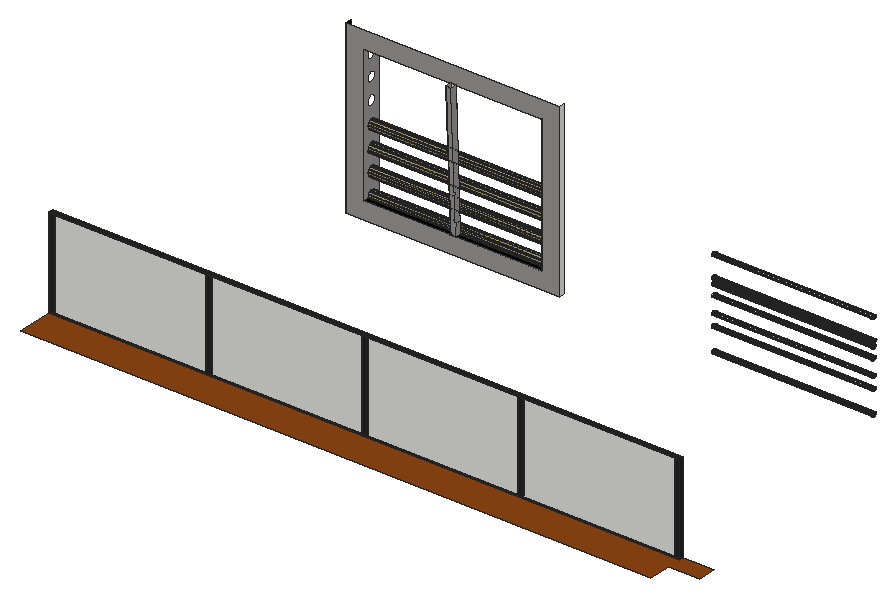
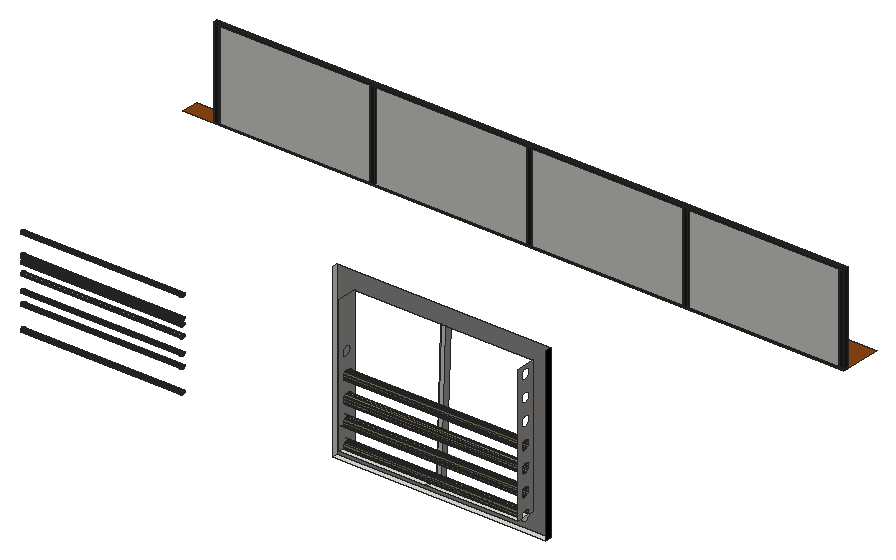
# SketchUp Ruby script. Lengths in inches.
U = 1.inch
M = Sketchup.active_model
def pt(a) = Geom::Point3d.new(a.map { |v| v * U })
def face(e, loops, mat)
  f = e.add_face(loops[0].map { |a| pt(a) })
  loops[1..].each { |l| e.add_face(l.map { |a| pt(a) }).erase! }
  f.material = f.back_material = mat if mat
  f
end
# faces: each face lists its corners as indices into pts; further lists are holes
def faces(e, pts, list, mat = nil) = list.each { |f| face(e, (f[0].is_a?(Array) ? f : [f]).map { |l| l.map { |i| pts[i] } }, mat) }
# xy, xz, yz: faces in a plane at the given z, y or x. An outline is a flat list of corners, or four numbers for a rectangle; further outlines are holes
def ring(l) = l.size == 4 ? [[l[0], l[1]], [l[2], l[1]], [l[2], l[3]], [l[0], l[3]]] : l.each_slice(2).to_a
def flat(e, list, mat, &to3) = list.each { |f| face(e, (f[0].is_a?(Array) ? f : [f]).map { |l| ring(l).map { |u, v| to3.(u, v) } }, mat) }
def xy(e, z, list, mat = nil) = flat(e, list, mat) { |x, y| [x, y, z] }
def xz(e, y, list, mat = nil) = flat(e, list, mat) { |x, z| [x, y, z] }
def yz(e, x, list, mat = nil) = flat(e, list, mat) { |y, z| [x, y, z] }
def lines(e, pts, list) = list.each { |a, b| e.add_line(pt(pts[a]), pt(pts[b])) }
# prism: a flat outline (further loops are holes) pulled along v
def prism(e, loops, v, mat = nil)
  f = face(e, loops, mat); d = Geom::Vector3d.new(v.map { |x| x * U })
  f.pushpull(f.normal.samedirection?(d) ? d.length : -d.length)
end
def box(e, o, s, mat = nil) = prism(e, [[o, [o[0] + s[0], o[1], o[2]], [o[0] + s[0], o[1] + s[1], o[2]], [o[0], o[1] + s[1], o[2]]]], [0, 0, s[2]], mat)
def at(x, y, z, deg = 0) = Geom::Transformation.translation(pt([x, y, z])) * Geom::Transformation.rotation(ORIGIN, Z_AXIS, deg.degrees)
def axes(o, x, y, z) = Geom::Transformation.new([*x, 0, *y, 0, *z, 0, *pt(o).to_a, 1])
def part(name) = M.definitions.add(name)
# library, detail: a bought-in or finely detailed component or shape, given as its bounding box
def library(name, o, s) = part(name).tap { |d| box(d.entities, o, s) }
def detail(e, o, s) = box(e.add_group.entities, o, s)
def put(e, d, t, mat = nil) = e.add_instance(d, t).tap { |i| i.material = mat if mat }
def group(e, t, mat = nil) = e.add_group.tap { |g| g.transformation = t; g.material = mat if mat }.entities
root = M.entities
M.materials.add("[0043_SaddleBrown]").color = [139, 69, 19]
M.materials.add("[0136_Charcoal]").color = [35, 35, 35]
M.materials.add("[Color M09]").color = [0, 0, 0]
M.materials.add("[Concrete Aggregate Smoke]").color = [154, 150, 148]
M.materials.add("[Terrazzo Tile Light]").color = [219, 217, 210]
M.materials.add("[Wood Lumber ButtJoined]").color = [164, 152, 112]
c1 = part("Group\#2")
box(c1.entities,[-152.36,0,0],[152.36,1.57,1.57])
c2 = part("Glass+Wall")
g1 = group(c2.entities,at(79.73,0,0))
g2 = group(g1,at(0,0,0))
g3 = group(g2,at(195.28,0,0),"[0136_Charcoal]")
box(g3,[-195.28,0,0],[195.28,1.57,1.57])
put(g2,c1,axes([1.57,0,116.54],[0,0,0.75452],[0,1,0],[-1,0,0]),"[0136_Charcoal]")
put(g2,c1,axes([50,0,116.54],[0,0,0.75452],[0,1,0],[-1,0,0]),"[0136_Charcoal]")
g4 = group(g2,at(195.28,0,115.75),"[0136_Charcoal]")
box(g4,[-195.28,0,0.79],[195.28,1.57,1.57])
put(g2,c1,axes([98.43,0,116.54],[0,0,0.75452],[0,1,0],[-1,0,0]),"[0136_Charcoal]")
put(g2,c1,axes([146.85,0,116.54],[0,0,0.75452],[0,1,0],[-1,0,0]),"[0136_Charcoal]")
put(g2,c1,axes([195.28,0,116.54],[0,0,0.75452],[0,1,0],[-1,0,0]),"[0136_Charcoal]")
g5 = group(g1,at(1.57,0.39,1.57))
box(g5,[0,0,0],[192.125,0.79,114.96])
xy(root,127.72,[[282.78,244.17,394.09,247.17]])
xy(root,136.72,[[291.78,246.86,291.78,251.79,338.43,251.79,338.43,247.17,339.9,247.17,339.9,251.79,385.09,251.79,385.09,246.86],[385.09,246.86,387.03,251.79],[338.43,247.17,339.9,251.79],[291.78,251.79,338.43,254.42],[338.43,251.79,339.9,254.42],
  [339.9,251.79,385.09,254.42]])
xy(root,136.72,[[291.78,244.17,385.09,246.86]],"[Color M09]")
xy(root,144,[[258.19,62.42,587.04,62.42,587.04,74.42,603,74.42,603,83.42,258.19,83.42]],"[0043_SaddleBrown]")
xz(root,244.17,[[[282.78,127.72,394.09,216.54],[291.78,136.72,385.09,207.54]]],"[Concrete Aggregate Smoke]")
yz(root,282.78,[[244.17,127.72,247.17,216.54]],"[Color M09]")
yz(root,291.78,[[249.32,134.85,249.99,134.94,250.6,135.2,251.14,135.6,251.54,136.13,251.79,136.72,246.86,136.72,247.1,136.13,247.51,135.6,248.04,135.2,248.66,134.94]])
yz(root,291.78,[[[244.17,136.72,246.86,136.72,246.85,136.75,246.76,137.42,246.85,138.08,247.1,138.7,247.51,139.23,248.04,139.63,248.66,139.89,249.32,139.98,249.99,139.89,250.6,139.63,251.14,139.23,251.54,138.7,251.8,138.08,251.89,137.42,251.8,136.75,251.79,136.72,254.42,136.72,254.42,207.54,244.17,207.54],[249.32,200.85,248.66,200.94,248.04,201.2,247.51,201.6,247.1,202.13,246.85,202.75,246.76,203.42,246.85,204.08,247.1,204.7,247.51,205.23,248.04,205.63,248.66,205.89,249.32,205.98,249.99,205.89,250.6,205.63,251.14,205.23,251.54,204.7,251.8,204.08,251.89,203.42,251.8,202.75,251.54,202.13,251.14,201.6,250.6,201.2,249.99,200.94],[249.32,189.85,248.66,189.94,248.04,190.2,247.51,190.6,247.1,191.13,246.85,191.75,246.76,192.42,246.85,193.08,247.1,193.7,247.51,194.23,248.04,194.63,248.66,194.89,249.32,194.98,249.99,194.89,250.6,194.63,251.14,194.23,251.54,193.7,251.8,193.08,251.89,192.42,251.8,191.75,251.54,191.13,251.14,190.6,250.6,190.2,249.99,189.94],[249.32,178.85,248.66,178.94,248.04,179.2,247.51,179.6,247.1,180.13,246.85,180.75,246.76,181.42,246.85,182.08,247.1,182.7,247.51,183.23,248.04,183.63,248.66,183.89,249.32,183.98,249.99,183.89,250.6,183.63,251.14,183.23,251.54,182.7,251.8,182.08,251.89,181.42,251.8,180.75,251.54,180.13,251.14,179.6,250.6,179.2,249.99,178.94],[249.32,167.85,248.66,167.94,248.04,168.2,247.51,168.6,247.1,169.13,246.85,169.75,246.76,170.42,246.85,171.08,247.1,171.7,247.51,172.23,248.04,172.63,248.66,172.89,249.32,172.98,249.99,172.89,250.6,172.63,251.14,172.23,251.54,171.7,251.8,171.08,251.89,170.42,251.8,169.75,251.54,169.13,251.14,168.6,250.6,168.2,249.99,167.94],[249.32,156.85,248.66,156.94,248.04,157.2,247.51,157.6,247.1,158.13,246.85,158.75,246.76,159.42,246.85,160.08,247.1,160.7,247.51,161.23,248.04,161.63,248.66,161.89,249.32,161.98,249.99,161.89,250.6,161.63,251.14,161.23,251.54,160.7,251.8,160.08,251.89,159.42,251.8,158.75,251.54,158.13,251.14,157.6,250.6,157.2,249.99,156.94],[249.32,145.85,248.66,145.94,248.04,146.2,247.51,146.6,247.1,147.13,246.85,147.75,246.76,148.42,246.85,149.08,247.1,149.7,247.51,150.23,248.04,150.63,248.66,150.89,249.32,150.98,249.99,150.89,250.6,150.63,251.14,150.23,251.54,149.7,251.8,149.08,251.89,148.42,251.8,147.75,251.54,147.13,251.14,146.6,250.6,146.2,249.99,145.94]]],"[Concrete Aggregate Smoke]")
yz(root,337.18,[[244.18,136.6,244.17,136.72,241.18,207.41,244.17,207.54,247.17,136.72]],"[Concrete Aggregate Smoke]")
yz(root,339.9,[[244.18,136.6,247.17,136.72,244.17,207.54,241.18,207.41,244.17,136.72]],"[Concrete Aggregate Smoke]")
yz(root,385.09,[[[244.17,136.72,254.42,207.54],[249.32,156.85,249.99,156.94,250.6,157.2,251.14,157.6,251.54,158.13,251.8,158.75,251.89,159.42,251.8,160.08,251.54,160.7,251.14,161.23,250.6,161.63,249.99,161.89,249.32,161.98,248.66,161.89,248.04,161.63,247.51,161.23,247.1,160.7,246.85,160.08,246.76,159.42,246.85,158.75,247.1,158.13,247.51,157.6,248.04,157.2,248.66,156.94],[249.32,167.85,249.99,167.94,250.6,168.2,251.14,168.6,251.54,169.13,251.8,169.75,251.89,170.42,251.8,171.08,251.54,171.7,251.14,172.23,250.6,172.63,249.99,172.89,249.32,172.98,248.66,172.89,248.04,172.63,247.51,172.23,247.1,171.7,246.85,171.08,246.76,170.42,246.85,169.75,247.1,169.13,247.51,168.6,248.04,168.2,248.66,167.94],[249.32,178.85,249.99,178.94,250.6,179.2,251.14,179.6,251.54,180.13,251.8,180.75,251.89,181.42,251.8,182.08,251.54,182.7,251.14,183.23,250.6,183.63,249.99,183.89,249.32,183.98,248.66,183.89,248.04,183.63,247.51,183.23,247.1,182.7,246.85,182.08,246.76,181.42,246.85,180.75,247.1,180.13,247.51,179.6,248.04,179.2,248.66,178.94]]],"[Concrete Aggregate Smoke]")
yz(root,386.78,[[249.32,145.85,249.99,145.94,250.6,146.2,251.14,146.6,251.54,147.13,251.8,147.75,251.89,148.42,251.8,149.08,251.54,149.7,251.14,150.23,250.6,150.63,249.99,150.89,249.32,150.98,248.66,150.89,248.04,150.63,247.51,150.23,247.1,149.7,246.85,149.08,246.76,148.42,246.85,147.75,247.1,147.13,247.51,146.6,248.04,146.2,248.66,145.94]])
yz(root,387.03,[[246.86,136.72,251.79,136.72,251.8,136.75,251.89,137.42,251.8,138.08,251.54,138.7,251.14,139.23,250.6,139.63,249.99,139.89,249.32,139.98,248.66,139.89,248.04,139.63,247.51,139.23,247.1,138.7,246.85,138.08,246.76,137.42,246.85,136.75]])
yz(root,394.09,[[244.17,127.72,247.17,216.54]])
p = [[473.23,245.22,128.58],[473.23,245.45,128.48],[557.23,245.45,128.48],[557.23,245.22,128.58],[473.23,245.69,128.45],[557.23,245.69,128.45],
  [473.23,245.94,128.48],[557.23,245.94,128.48],[473.23,246.16,128.58],[557.23,246.16,128.58],[473.23,245.03,128.73],[557.23,245.03,128.73],
  [473.23,246.36,128.73],[557.23,246.36,128.73],[473.23,244.88,128.92],[557.23,244.88,128.92],[473.23,246.5,128.92],[557.23,246.5,128.92],
  [473.23,244.79,129.15],[557.23,244.79,129.15],[473.23,246.6,129.15],[557.23,246.6,129.15],[473.23,244.75,129.39],[557.23,244.75,129.39],
  [473.23,246.63,129.39],[557.23,246.63,129.39],[473.23,244.79,129.63],[557.23,244.79,129.63],[473.23,246.6,129.63],[557.23,246.6,129.63],
  [473.23,244.88,129.86],[557.23,244.88,129.86],[473.23,246.5,129.86],[557.23,246.5,129.86],[473.23,245.03,130.05],[557.23,245.03,130.05],
  [473.23,246.36,130.05],[557.23,246.36,130.05],[473.23,245.22,130.2],[557.23,245.22,130.2],[473.23,246.16,130.2],[557.23,246.16,130.2],
  [473.23,245.45,130.29],[557.23,245.45,130.29],[473.23,245.94,130.29],[557.23,245.94,130.29],[473.23,245.69,130.33],[557.23,245.69,130.33],
  [338.43,247.17,136.72],[339.9,247.17,136.72],[339.9,244.18,136.6],[337.18,244.18,136.6],[337.18,247.17,136.72],[339.9,244.17,136.72],
  [338.43,244.17,136.72],[337.18,244.17,136.72],[339.9,241.18,207.41],[337.18,241.18,207.41],[337.18,244.17,207.54],[338.43,244.17,207.54],
  [339.9,244.17,207.54],[291.78,246.85,136.75],[291.78,246.86,136.72],[385.09,246.86,136.72],[387.03,246.86,136.72],[387.03,246.85,136.75],
  [291.78,251.79,136.72],[291.78,251.8,136.75],[387.03,251.8,136.75],[387.03,251.79,136.72],[385.09,251.79,136.72],[339.9,251.79,136.72],
  [338.43,251.79,136.72],[291.78,246.76,137.42],[387.03,246.76,137.42],[291.78,251.89,137.42],[387.03,251.89,137.42],[291.78,246.85,138.08],
  [387.03,246.85,138.08],[291.78,251.8,138.08],[387.03,251.8,138.08],[291.78,247.1,138.7],[387.03,247.1,138.7],[291.78,251.54,138.7],
  [387.03,251.54,138.7],[291.78,247.51,139.23],[387.03,247.51,139.23],[291.78,251.14,139.23],[387.03,251.14,139.23],[291.78,248.04,139.63],
  [387.03,248.04,139.63],[291.78,250.6,139.63],[387.03,250.6,139.63],[291.78,248.66,139.89],[387.03,248.66,139.89],[291.78,249.99,139.89],
  [387.03,249.99,139.89],[291.78,249.32,139.98],[387.03,249.32,139.98],[473.23,245.22,140.58],[473.23,245.45,140.48],[557.23,245.45,140.48],
  [557.23,245.22,140.58],[473.23,245.69,140.45],[557.23,245.69,140.45],[473.23,245.94,140.48],[557.23,245.94,140.48],[473.23,246.16,140.58],
  [557.23,246.16,140.58],[473.23,245.03,140.73],[557.23,245.03,140.73],[473.23,246.36,140.73],[557.23,246.36,140.73],[473.23,244.88,140.92],
  [557.23,244.88,140.92],[473.23,246.5,140.92],[557.23,246.5,140.92],[473.23,244.79,141.15],[557.23,244.79,141.15],[473.23,246.6,141.15],
  [557.23,246.6,141.15],[473.23,244.75,141.39],[557.23,244.75,141.39],[473.23,246.63,141.39],[557.23,246.63,141.39],[473.23,244.79,141.63],
  [557.23,244.79,141.63],[473.23,246.6,141.63],[557.23,246.6,141.63],[473.23,244.88,141.86],[557.23,244.88,141.86],[473.23,246.5,141.86],
  [557.23,246.5,141.86],[473.23,245.03,142.05],[557.23,245.03,142.05],[473.23,246.36,142.05],[557.23,246.36,142.05],[473.23,245.22,142.2],
  [557.23,245.22,142.2],[473.23,246.16,142.2],[557.23,246.16,142.2],[473.23,245.45,142.29],[557.23,245.45,142.29],[473.23,245.94,142.29],
  [557.23,245.94,142.29],[473.23,245.69,142.33],[557.23,245.69,142.33],[291.78,248.04,146.2],[291.78,248.66,145.94],[386.78,248.66,145.94],
  [386.78,248.04,146.2],[291.78,249.32,145.85],[386.78,249.32,145.85],[291.78,249.99,145.94],[386.78,249.99,145.94],[291.78,250.6,146.2],
  [386.78,250.6,146.2],[291.78,247.51,146.6],[386.78,247.51,146.6],[291.78,251.14,146.6],[386.78,251.14,146.6],[473.23,245.22,146.58],
  [473.23,245.45,146.48],[557.23,245.45,146.48],[557.23,245.22,146.58],[473.23,245.69,146.45],[557.23,245.69,146.45],[473.23,245.94,146.48],
  [557.23,245.94,146.48],[473.23,246.16,146.58],[557.23,246.16,146.58],[473.23,245.03,146.73],[557.23,245.03,146.73],[473.23,246.36,146.73],
  [557.23,246.36,146.73],[291.78,247.1,147.13],[386.78,247.1,147.13],[291.78,251.54,147.13],[386.78,251.54,147.13],[473.23,244.88,146.92],
  [557.23,244.88,146.92],[473.23,246.5,146.92],[557.23,246.5,146.92],[473.23,244.79,147.15],[557.23,244.79,147.15],[473.23,246.6,147.15],
  [557.23,246.6,147.15],[473.23,244.75,147.39],[557.23,244.75,147.39],[473.23,246.63,147.39],[557.23,246.63,147.39],[291.78,246.85,147.75],
  [386.78,246.85,147.75],[291.78,251.8,147.75],[386.78,251.8,147.75],[473.23,244.79,147.63],[557.23,244.79,147.63],[473.23,246.6,147.63],
  [557.23,246.6,147.63],[473.23,244.88,147.86],[557.23,244.88,147.86],[473.23,246.5,147.86],[557.23,246.5,147.86],[291.78,246.76,148.42],
  [386.78,246.76,148.42],[291.78,251.89,148.42],[386.78,251.89,148.42],[473.23,245.03,148.05],[557.23,245.03,148.05],[473.23,246.36,148.05],
  [557.23,246.36,148.05],[473.23,245.22,148.2],[557.23,245.22,148.2],[473.23,246.16,148.2],[557.23,246.16,148.2],[473.23,245.45,148.29],
  [557.23,245.45,148.29],[473.23,245.94,148.29],[557.23,245.94,148.29],[473.23,245.69,148.33],[557.23,245.69,148.33],[291.78,246.85,149.08],
  [386.78,246.85,149.08],[291.78,251.8,149.08],[386.78,251.8,149.08],[291.78,247.1,149.7],[386.78,247.1,149.7],[291.78,251.54,149.7],
  [386.78,251.54,149.7],[291.78,247.51,150.23],[386.78,247.51,150.23],[291.78,251.14,150.23],[386.78,251.14,150.23],[291.78,248.04,150.63],
  [386.78,248.04,150.63],[291.78,250.6,150.63],[386.78,250.6,150.63],[291.78,248.66,150.89],[386.78,248.66,150.89],[291.78,249.99,150.89],
  [386.78,249.99,150.89],[291.78,249.32,150.98],[386.78,249.32,150.98],[473.23,245.22,154.83],[473.23,245.45,154.73],[557.23,245.45,154.73],
  [557.23,245.22,154.83],[473.23,245.69,154.7],[557.23,245.69,154.7],[473.23,245.94,154.73],[557.23,245.94,154.73],[473.23,246.16,154.83],
  [557.23,246.16,154.83],[473.23,245.03,154.98],[557.23,245.03,154.98],[473.23,246.36,154.98],[557.23,246.36,154.98],[473.23,244.88,155.17],
  [557.23,244.88,155.17],[473.23,246.5,155.17],[557.23,246.5,155.17],[473.23,244.79,155.4],[557.23,244.79,155.4],[473.23,246.6,155.4],
  [557.23,246.6,155.4],[473.23,244.75,155.64],[557.23,244.75,155.64],[473.23,246.63,155.64],[557.23,246.63,155.64],[473.23,244.79,155.88],
  [557.23,244.79,155.88],[473.23,246.6,155.88],[557.23,246.6,155.88],[473.23,244.88,156.11],[557.23,244.88,156.11],[473.23,246.5,156.11],
  [557.23,246.5,156.11],[473.23,245.03,156.3],[557.23,245.03,156.3],[473.23,246.36,156.3],[557.23,246.36,156.3],[473.23,245.22,156.45],
  [557.23,245.22,156.45],[473.23,246.16,156.45],[557.23,246.16,156.45],[473.23,245.45,156.54],[557.23,245.45,156.54],[473.23,245.69,156.58],
  [557.23,245.69,156.58],[473.23,245.94,156.54],[557.23,245.94,156.54],[291.78,248.04,157.2],[291.78,248.66,156.94],[385.09,248.66,156.94],
  [385.09,248.04,157.2],[291.78,249.32,156.85],[385.09,249.32,156.85],[291.78,249.99,156.94],[385.09,249.99,156.94],[291.78,250.6,157.2],
  [385.09,250.6,157.2],[291.78,247.51,157.6],[385.09,247.51,157.6],[291.78,251.14,157.6],[385.09,251.14,157.6],[291.78,247.1,158.13],
  [385.09,247.1,158.13],[291.78,251.54,158.13],[385.09,251.54,158.13],[291.78,246.85,158.75],[385.09,246.85,158.75],[291.78,251.8,158.75],
  [385.09,251.8,158.75],[291.78,246.76,159.42],[385.09,246.76,159.42],[291.78,251.89,159.42],[385.09,251.89,159.42],[291.78,246.85,160.08],
  [385.09,246.85,160.08],[291.78,251.8,160.08],[385.09,251.8,160.08],[291.78,247.1,160.7],[385.09,247.1,160.7],[291.78,251.54,160.7],
  [385.09,251.54,160.7],[473.23,245.22,160.33],[473.23,245.45,160.23],[557.23,245.45,160.23],[557.23,245.22,160.33],[473.23,245.69,160.2],
  [557.23,245.69,160.2],[473.23,245.94,160.23],[557.23,245.94,160.23],[473.23,246.16,160.33],[557.23,246.16,160.33],[473.23,245.03,160.48],
  [557.23,245.03,160.48],[473.23,246.36,160.48],[557.23,246.36,160.48],[473.23,244.88,160.67],[557.23,244.88,160.67],[473.23,246.5,160.67],
  [557.23,246.5,160.67],[473.23,244.79,160.9],[557.23,244.79,160.9],[473.23,246.6,160.9],[557.23,246.6,160.9],[291.78,247.51,161.23],
  [385.09,247.51,161.23],[291.78,251.14,161.23],[385.09,251.14,161.23],[473.23,244.75,161.14],[557.23,244.75,161.14],[473.23,246.63,161.14],
  [557.23,246.63,161.14],[473.23,244.79,161.38],[557.23,244.79,161.38],[473.23,246.6,161.38],[557.23,246.6,161.38],[291.78,248.04,161.63],
  [385.09,248.04,161.63],[291.78,250.6,161.63],[385.09,250.6,161.63],[473.23,244.88,161.61],[557.23,244.88,161.61],[473.23,246.5,161.61],
  [557.23,246.5,161.61],[473.23,245.03,161.8],[557.23,245.03,161.8],[473.23,246.36,161.8],[557.23,246.36,161.8],[291.78,248.66,161.89],
  [385.09,248.66,161.89],[291.78,249.99,161.89],[385.09,249.99,161.89],[473.23,245.22,161.95],[557.23,245.22,161.95],[473.23,246.16,161.95],
  [557.23,246.16,161.95],[291.78,249.32,161.98],[385.09,249.32,161.98],[473.23,245.45,162.04],[557.23,245.45,162.04],[473.23,245.69,162.08],
  [557.23,245.69,162.08],[473.23,245.94,162.04],[557.23,245.94,162.04],[473.23,245.22,163.08],[473.23,245.45,162.98],[557.42,245.45,162.98],
  [557.42,245.22,163.08],[473.23,245.69,162.95],[557.42,245.69,162.95],[473.23,245.94,162.98],[557.42,245.94,162.98],[473.23,246.16,163.08],
  [557.42,246.16,163.08],[473.23,245.03,163.23],[557.42,245.03,163.23],[473.23,246.36,163.23],[557.42,246.36,163.23],[473.23,244.88,163.42],
  [557.42,244.88,163.42],[473.23,246.5,163.42],[557.42,246.5,163.42],[473.23,244.79,163.65],[557.42,244.79,163.65],[473.23,246.6,163.65],
  [557.42,246.6,163.65],[473.23,244.75,163.89],[557.42,244.75,163.89],[473.23,246.63,163.89],[557.42,246.63,163.89],[473.23,244.79,164.13],
  [557.42,244.79,164.13],[473.23,246.6,164.13],[557.42,246.6,164.13],[473.23,244.88,164.36],[557.42,244.88,164.36],[473.23,246.5,164.36],
  [557.42,246.5,164.36],[473.23,245.03,164.55],[557.42,245.03,164.55],[473.23,246.36,164.55],[557.42,246.36,164.55],[473.23,245.22,164.7],
  [557.42,245.22,164.7],[473.23,246.16,164.7],[557.42,246.16,164.7],[473.23,245.45,164.79],[557.42,245.45,164.79],[473.23,245.94,164.79],
  [557.42,245.94,164.79],[473.23,245.69,164.83],[557.42,245.69,164.83],[291.78,248.04,168.2],[291.78,248.66,167.94],[385.09,248.66,167.94],
  [385.09,248.04,168.2],[291.78,249.32,167.85],[385.09,249.32,167.85],[291.78,249.99,167.94],[385.09,249.99,167.94],[291.78,250.6,168.2],
  [385.09,250.6,168.2],[291.78,247.51,168.6],[385.09,247.51,168.6],[291.78,251.14,168.6],[385.09,251.14,168.6],[291.78,247.1,169.13],
  [385.09,247.1,169.13],[291.78,251.54,169.13],[385.09,251.54,169.13],[291.78,246.85,169.75],[385.09,246.85,169.75],[291.78,251.8,169.75],
  [385.09,251.8,169.75],[291.78,246.76,170.42],[385.09,246.76,170.42],[291.78,251.89,170.42],[385.09,251.89,170.42],[291.78,246.85,171.08],
  [385.09,246.85,171.08],[291.78,251.8,171.08],[385.09,251.8,171.08],[291.78,247.1,171.7],[385.09,247.1,171.7],[291.78,251.54,171.7],
  [385.09,251.54,171.7],[291.78,247.51,172.23],[385.09,247.51,172.23],[291.78,251.14,172.23],[385.09,251.14,172.23],[291.78,248.04,172.63],
  [385.09,248.04,172.63],[291.78,250.6,172.63],[385.09,250.6,172.63],[291.78,248.66,172.89],[385.09,248.66,172.89],[291.78,249.99,172.89],
  [385.09,249.99,172.89],[291.78,249.32,172.98],[385.09,249.32,172.98],[473.23,245.22,174.08],[473.23,245.45,173.98],[557.23,245.45,173.98],
  [557.23,245.22,174.08],[473.23,245.69,173.95],[557.23,245.69,173.95],[473.23,245.94,173.98],[557.23,245.94,173.98],[473.23,246.16,174.08],
  [557.23,246.16,174.08],[473.23,245.03,174.23],[557.23,245.03,174.23],[473.23,246.36,174.23],[557.23,246.36,174.23],[473.23,244.88,174.42],
  [557.23,244.88,174.42],[473.23,246.5,174.42],[557.23,246.5,174.42],[473.23,244.79,174.65],[557.23,244.79,174.65],[473.23,246.6,174.65],
  [557.23,246.6,174.65],[473.23,244.75,174.89],[557.23,244.75,174.89],[473.23,246.63,174.89],[557.23,246.63,174.89],[473.23,244.79,175.13],
  [557.23,244.79,175.13],[473.23,246.6,175.13],[557.23,246.6,175.13],[473.23,244.88,175.36],[557.23,244.88,175.36],[473.23,246.5,175.36],
  [557.23,246.5,175.36],[473.23,245.03,175.55],[557.23,245.03,175.55],[473.23,246.36,175.55],[557.23,246.36,175.55],[473.23,245.22,175.7],
  [557.23,245.22,175.7],[473.23,246.16,175.7],[557.23,246.16,175.7],[473.23,245.45,175.79],[557.23,245.45,175.79],[473.23,245.94,175.79],
  [557.23,245.94,175.79],[473.23,245.69,175.83],[557.23,245.69,175.83]]
faces(root,p,[[0,1,2,3],[1,4,5,2],[4,6,7,5],[6,8,9,7],[10,0,3,11],[8,12,13,9],[14,10,11,15],[12,16,17,13],
  [18,14,15,19],[16,20,21,17],[22,18,19,23],[20,24,25,21],[26,22,23,27],[24,28,29,25],[30,26,27,31],[28,32,33,29],
  [34,30,31,35],[32,36,37,33],[38,34,35,39],[36,40,41,37],[42,38,39,43],[40,44,45,41],[46,42,43,47],[44,46,47,45],
  [99,100,101,102],[100,103,104,101],[103,105,106,104],[105,107,108,106],[109,99,102,110],[107,111,112,108],[113,109,110,114],[111,115,116,112],
  [117,113,114,118],[115,119,120,116],[121,117,118,122],[119,123,124,120],[125,121,122,126],[123,127,128,124],[129,125,126,130],[127,131,132,128],
  [133,129,130,134],[131,135,136,132],[137,133,134,138],[135,139,140,136],[141,137,138,142],[139,143,144,140],[145,141,142,146],[143,145,146,144],
  [161,162,163,164],[162,165,166,163],[165,167,168,166],[167,169,170,168],[171,161,164,172],[169,173,174,170],[179,171,172,180],[173,181,182,174],
  [183,179,180,184],[181,185,186,182],[187,183,184,188],[185,189,190,186],[195,187,188,196],[189,197,198,190],[199,195,196,200],[197,201,202,198],
  [207,199,200,208],[201,209,210,202],[211,207,208,212],[209,213,214,210],[215,211,212,216],[213,217,218,214],[219,215,216,220],[217,219,220,218],
  [243,244,245,246],[244,247,248,245],[247,249,250,248],[249,251,252,250],[253,243,246,254],[251,255,256,252],[257,253,254,258],[255,259,260,256],
  [261,257,258,262],[259,263,264,260],[265,261,262,266],[263,267,268,264],[269,265,266,270],[267,271,272,268],[273,269,270,274],[271,275,276,272],
  [277,273,274,278],[275,279,280,276],[281,277,278,282],[279,283,284,280],[285,281,282,286],[287,285,286,288],[289,287,288,290],[283,289,290,284],
  [325,326,327,328],[326,329,330,327],[329,331,332,330],[331,333,334,332],[335,325,328,336],[333,337,338,334],[339,335,336,340],[337,341,342,338],
  [343,339,340,344],[341,345,346,342],[351,343,344,352],[345,353,354,346],[355,351,352,356],[353,357,358,354],[363,355,356,364],[357,365,366,358],
  [367,363,364,368],[365,369,370,366],[375,367,368,376],[369,377,378,370],[381,375,376,382],[383,381,382,384],[385,383,384,386],[377,385,386,378],
  [387,388,389,390],[388,391,392,389],[391,393,394,392],[393,395,396,394],[397,387,390,398],[395,399,400,396],[401,397,398,402],[399,403,404,400],
  [405,401,402,406],[403,407,408,404],[409,405,406,410],[407,411,412,408],[413,409,410,414],[411,415,416,412],[417,413,414,418],[415,419,420,416],
  [421,417,418,422],[419,423,424,420],[425,421,422,426],[423,427,428,424],[429,425,426,430],[427,431,432,428],[431,433,434,432],[483,484,485,486],
  [484,487,488,485],[487,489,490,488],[489,491,492,490],[493,483,486,494],[491,495,496,492],[497,493,494,498],[495,499,500,496],[501,497,498,502],
  [499,503,504,500],[505,501,502,506],[503,507,508,504],[509,505,506,510],[507,511,512,508],[513,509,510,514],[511,515,516,512],[517,513,514,518],
  [515,519,520,516],[521,517,518,522],[519,523,524,520],[525,521,522,526],[523,527,528,524],[529,525,526,530],[527,529,530,528]],"[Terrazzo Tile Light]")
faces(root,p,[[48,49,50,51,52],[50,53,54,55,51],[49,48,52,58,59,60]])
faces(root,p,[[56,57,55,54,53]],"[Concrete Aggregate Smoke]")
faces(root,p,[[61,62,63,64,65],[66,67,68,69,70,71,72],[73,61,65,74],[67,75,76,68],[77,73,74,78],[75,79,80,76],[81,77,78,82],[79,83,84,80],
  [85,81,82,86],[83,87,88,84],[89,85,86,90],[87,91,92,88],[93,89,90,94],[91,95,96,92],[97,93,94,98],[95,97,98,96],
  [147,148,149,150],[148,151,152,149],[151,153,154,152],[153,155,156,154],[157,147,150,158],[155,159,160,156],[175,157,158,176],[159,177,178,160],
  [191,175,176,192],[177,193,194,178],[203,191,192,204],[193,205,206,194],[221,203,204,222],[205,223,224,206],[225,221,222,226],[223,227,228,224],
  [229,225,226,230],[227,231,232,228],[233,229,230,234],[231,235,236,232],[237,233,234,238],[235,239,240,236],[241,237,238,242],[239,241,242,240],
  [291,292,293,294],[292,295,296,293],[295,297,298,296],[297,299,300,298],[301,291,294,302],[299,303,304,300],[305,301,302,306],[303,307,308,304],
  [309,305,306,310],[307,311,312,308],[313,309,310,314],[311,315,316,312],[317,313,314,318],[315,319,320,316],[321,317,318,322],[319,323,324,320],
  [347,321,322,348],[323,349,350,324],[359,347,348,360],[349,361,362,350],[371,359,360,372],[361,373,374,362],[379,371,372,380],[373,379,380,374],
  [435,436,437,438],[436,439,440,437],[439,441,442,440],[441,443,444,442],[445,435,438,446],[443,447,448,444],[449,445,446,450],[447,451,452,448],
  [453,449,450,454],[451,455,456,452],[457,453,454,458],[455,459,460,456],[461,457,458,462],[459,463,464,460],[465,461,462,466],[463,467,468,464],
  [469,465,466,470],[467,471,472,468],[473,469,470,474],[471,475,476,472],[477,473,474,478],[475,479,480,476],[481,477,478,482],[479,481,482,480]],"[Wood Lumber ButtJoined]")
put(root,c2,axes([123.93,83.42,144],[1.68404,0,0],[0,-1.352,0],[0,0,0.4]))
